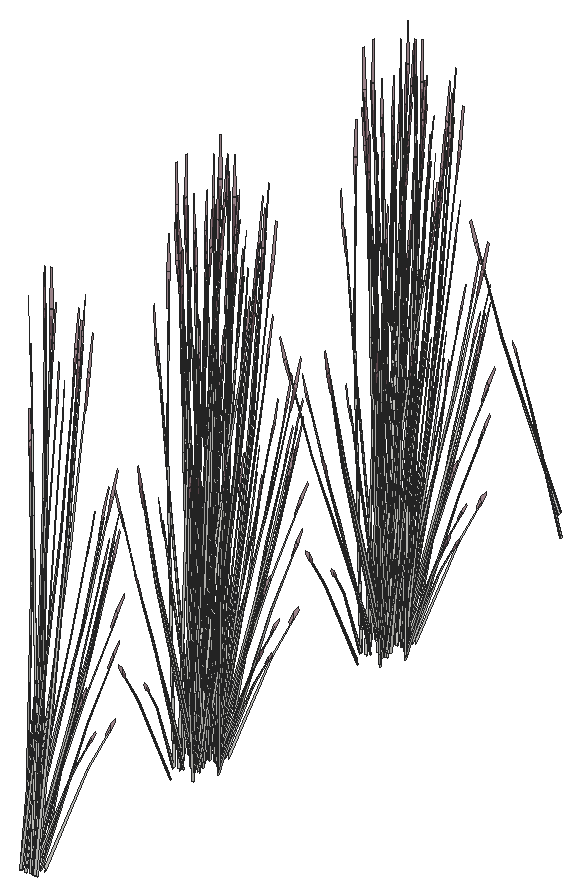
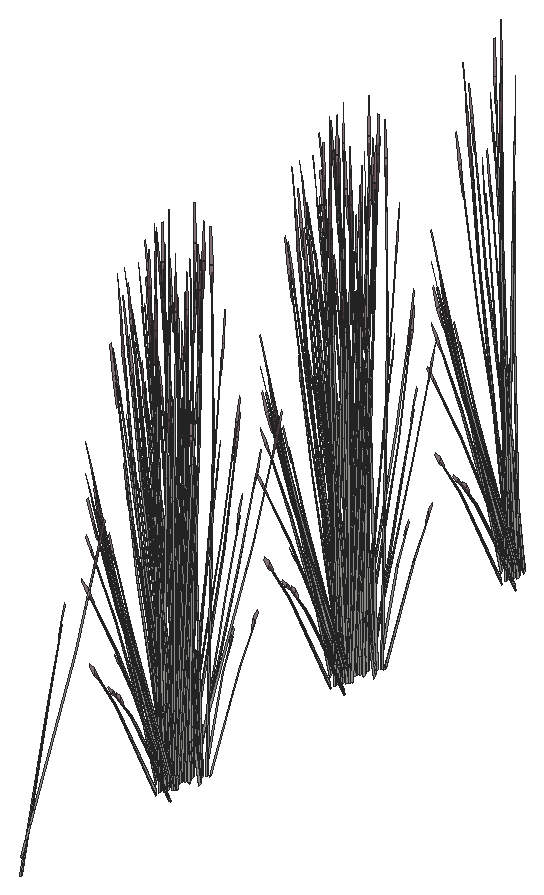
# SketchUp Ruby script. Lengths in inches.
U = 1.inch
M = Sketchup.active_model
def pt(a) = Geom::Point3d.new(a.map { |v| v * U })
def face(e, loops, mat)
  f = e.add_face(loops[0].map { |a| pt(a) })
  loops[1..].each { |l| e.add_face(l.map { |a| pt(a) }).erase! }
  f.material = f.back_material = mat if mat
  f
end
# faces: each face lists its corners as indices into pts; further lists are holes
def faces(e, pts, list, mat = nil) = list.each { |f| face(e, (f[0].is_a?(Array) ? f : [f]).map { |l| l.map { |i| pts[i] } }, mat) }
# xy, xz, yz: faces in a plane at the given z, y or x. An outline is a flat list of corners, or four numbers for a rectangle; further outlines are holes
def ring(l) = l.size == 4 ? [[l[0], l[1]], [l[2], l[1]], [l[2], l[3]], [l[0], l[3]]] : l.each_slice(2).to_a
def flat(e, list, mat, &to3) = list.each { |f| face(e, (f[0].is_a?(Array) ? f : [f]).map { |l| ring(l).map { |u, v| to3.(u, v) } }, mat) }
def xy(e, z, list, mat = nil) = flat(e, list, mat) { |x, y| [x, y, z] }
def xz(e, y, list, mat = nil) = flat(e, list, mat) { |x, z| [x, y, z] }
def yz(e, x, list, mat = nil) = flat(e, list, mat) { |y, z| [x, y, z] }
def lines(e, pts, list) = list.each { |a, b| e.add_line(pt(pts[a]), pt(pts[b])) }
# prism: a flat outline (further loops are holes) pulled along v
def prism(e, loops, v, mat = nil)
  f = face(e, loops, mat); d = Geom::Vector3d.new(v.map { |x| x * U })
  f.pushpull(f.normal.samedirection?(d) ? d.length : -d.length)
end
def box(e, o, s, mat = nil) = prism(e, [[o, [o[0] + s[0], o[1], o[2]], [o[0] + s[0], o[1] + s[1], o[2]], [o[0], o[1] + s[1], o[2]]]], [0, 0, s[2]], mat)
def at(x, y, z, deg = 0) = Geom::Transformation.translation(pt([x, y, z])) * Geom::Transformation.rotation(ORIGIN, Z_AXIS, deg.degrees)
def axes(o, x, y, z) = Geom::Transformation.new([*x, 0, *y, 0, *z, 0, *pt(o).to_a, 1])
def part(name) = M.definitions.add(name)
# library, detail: a bought-in or finely detailed component or shape, given as its bounding box
def library(name, o, s) = part(name).tap { |d| box(d.entities, o, s) }
def detail(e, o, s) = box(e.add_group.entities, o, s)
def put(e, d, t, mat = nil) = e.add_instance(d, t).tap { |i| i.material = mat if mat }
def group(e, t, mat = nil) = e.add_group.tap { |g| g.transformation = t; g.material = mat if mat }.entities
root = M.entities
M.materials.add("LightPink_Translucent").color = [144, 107, 117]
M.materials["LightPink_Translucent"].alpha = 0.75
c1 = part("blade")
p = [[2.15,0.21,22],[0,0.17,0],[0.09,0.45,0],[2.18,0.31,22],[2.29,0.31,22],[0.38,0.45,0],
  [2.48,0.24,33],[2.49,0.24,33],[2.48,0.22,33]]
faces(c1.entities,p,[[0,1,2,3],[4,5,2,3],[6,3,4,7],[8,0,3,6]])
c2 = part("seeds")
p = [[0.3,-0.1,1.38],[-0.01,-0.03,1.59],[-0.01,-0.03,0.03],[0.14,-0.07,-0.07],[0.29,-0.03,3],[0.15,0.01,3.11]]
faces(c2.entities,p,[[0,1,2,3],[1,0,4,5]],"LightPink_Translucent")
c3 = part("blade with seeds")
put(c3.entities,c1,at(0,0,0))
put(c3.entities,c2,axes([2.4,0.25,30.99],[1.5799,-0.05474,1.17369],[-0.12525,1.92788,0.29478],[-0.07173,-0.02425,1.56792]))
put(root,c3,axes([434.57,69.42,0.23],[-0.09062,-0.13571,1.22981],[0.11791,-0.44895,-0.26449],[0.18335,0.06082,0.52581]))
put(root,c3,axes([432.95,69.91,-0.1],[0.37935,0.24773,0],[-0.18257,0.51475,0],[0,0,1.5046]))
put(root,c3,axes([433.02,69.12,0.25],[0.278,0.33153,0.12452],[-0.23189,0.37404,-0.35559],[-0.06454,0.05057,1.09]))
put(root,c3,axes([433.74,69.69,2.28],[0.37615,0.01329,-0.61099],[-0.02526,0.55946,0.07373],[0.15935,0.05904,0.8643]))
put(root,c3,axes([433.32,70.14,0.13],[0.35217,-0.2759,0.427],[0.2105,0.49473,0],[-0.08021,0.06284,1.35453]))
put(root,c3,axes([432.81,69.7,-0.03],[0.1636,0.63392,-0.05171],[-0.46745,0.22213,0],[0.00571,0.02214,1.48069]))
put(root,c3,axes([434.35,68.56,0.04],[0.47052,0,0],[0,0.61671,-0.44382],[0,0.14046,1.40792]))
put(root,c3,axes([434.17,68.87,-0.11],[-0.47029,-0.00441,-0.0428],[0,-0.61671,0.42951],[-0.01478,0.14039,1.36183]))
put(root,c3,axes([433.15,68.34,0.29],[0.42377,0.26329,-0.25022],[-0.20405,0.55571,-0.43002],[0.01332,0.13644,1.37348]))
put(root,c3,axes([433.97,69.92,1.89],[0.2141,0.34548,-0.30456],[-0.24447,0.32704,0.39319],[0.12421,0.04976,0.75234]))
put(root,c3,axes([434.07,68.96,-0.26],[-0.26266,0.34428,-0.26641],[-0.26266,-0.34428,0.26641],[0,0.11089,1.19518]))
put(root,c3,axes([433.1,68.75,-0.1],[-0.18257,0.49721,-0.38476],[-0.37935,-0.23929,0.18517],[0,0.11462,1.23533]))
put(root,c3,axes([433.11,70.17,0],[0.47108,0.17935,0.2645],[-0.11785,0.64108,-0.31383],[-0.07797,0.08023,1.41801]))
put(root,c3,axes([434.25,68.97,-0.26],[0,0.5518,-0.427],[-0.42099,0,0],[0,0.12568,1.35453]))
put(root,c3,axes([433.71,70.12,0.38],[-0.21187,-0.15866,0.9878],[0.27357,-0.16121,0.72577],[0.07379,0.13656,0.21757]))
put(root,c3,axes([433.4,70.52,0.04],[0.23526,0.55293,0],[-0.3936,0.30836,-0.44382],[-0.08964,0.07023,1.40792]))
put(root,c3,axes([433.77,70.71,-0.72],[0.02741,-0.07966,1.51654],[0.34514,-0.23462,-0.23168],[0.10464,0.12143,0.25832]))
put(root,c3,axes([433.32,68.9,-0.2],[0.13798,0.50522,-0.59522],[-0.39745,0.18195,-0.15622],[0.01525,0.17108,1.31385]))
put(root,c3,axes([433.24,70.34,2.03],[0.37131,-0.13117,-0.43945],[0.06495,0.49674,-0.34039],[0.09973,0.14235,0.84085]))
put(root,c3,axes([433.75,70.84,0.29],[-0.2413,-0.01731,0.90352],[0.15935,-0.36755,0.49885],[0.09532,0.13058,0.70873]))
put(root,c3,axes([432.96,69.95,0.23],[0.00664,-0.18292,1.22981],[0.31732,-0.20432,-0.26449],[0.09796,0.21893,0.52581]))
put(root,c3,axes([432.16,70.69,-0.72],[0.0609,-0.03003,1.51654],[0.36632,0.16527,-0.23168],[0.01071,0.18627,0.25832]))
put(root,c3,axes([432.41,70.57,2.03],[0.3699,0.13833,-0.43945],[-0.12679,0.47426,-0.34039],[0.03392,0.19095,0.84085]))
put(root,c3,axes([432.24,70.86,1.89],[-0.11344,0.42434,-0.30456],[-0.33096,-0.12377,0.39319],[0.03035,0.17085,0.75234]))
put(root,c3,axes([432.28,70.48,2.28],[0.17959,0.44867,-0.61099],[-0.36969,0.25004,0.07373],[0.042,0.21679,0.8643]))
put(root,c3,axes([433.22,89.07,0.23],[-0.10696,0.11169,1.22981],[-0.32033,-0.19549,-0.26449],[0.05938,-0.24312,0.52581]))
put(root,c3,axes([432.43,88.47,-0.72],[-0.06312,0.01988,1.51654],[-0.34903,-0.22379,-0.23168],[0.00586,-0.18666,0.25832]))
put(root,c3,axes([433.48,89.9,2.28],[0.00979,-0.51041,-0.61099],[0.4123,0.03428,0.07373],[0.04351,-0.21623,0.8643]))
put(root,c3,axes([432.77,89.08,1.89],[0.11344,-0.42434,-0.30456],[0.33096,0.12377,0.39319],[-0.03035,-0.17085,0.75234]))
put(root,c3,axes([432.83,88.18,0.38],[0.04827,0.32177,0.9878],[-0.26778,-0.17821,0.72577],[0.02882,-0.16476,0.21757]))
put(root,c3,axes([433.4,89.73,2.03],[-0.26937,-0.37076,-0.43945],[0.28456,-0.3247,-0.34039],[0.04099,-0.18838,0.84085]))
put(root,c3,axes([433.65,89.59,1.89],[0.2546,-0.29052,-0.30456],[0.24101,0.33173,0.39319],[0.03667,-0.16855,0.75234]))
put(root,c3,axes([433.97,89.42,-0.72],[-0.05632,-0.04347,1.51654],[-0.14467,-0.48565,-0.23168],[0.09759,-0.13179,0.25832]))
put(root,c3,axes([433.97,90.79,2.28],[0.19655,-0.43539,-0.61099],[0.34443,0.30942,0.07373],[0.11736,-0.15774,0.8643]))
put(root,c3,axes([431.84,89.52,0.04],[-0.23526,-0.55293,0],[0.3936,-0.30836,-0.44382],[0.08964,-0.07023,1.40792]))
put(root,c3,axes([433.96,90.58,2.03],[-0.09666,-0.50384,-0.43945],[0.36608,-0.08814,-0.34039],[0.10491,-0.13533,0.84085]))
put(root,c3,axes([432.16,89.43,-0.26],[0.35217,-0.2759,-0.427],[0.2105,0.49473,0],[0.08021,-0.06284,1.35453]))
put(root,c3,axes([434.25,90.39,0.23],[-0.13443,-0.01634,1.22981],[-0.13772,-0.43844,-0.26449],[0.16514,-0.12403,0.52581]))
put(root,c3,axes([432.58,90.57,-0.23],[0.25345,-0.41475,-0.53624],[0.31485,0.37608,-0.14074],[0.10156,-0.10346,1.18365]))
put(root,c3,axes([434.41,89.58,0.38],[-0.12533,0.28089,0.9878],[-0.10773,-0.37739,0.72577],[0.10352,-0.09457,0.21757]))
put(root,c3,axes([434.23,90.64,1.89],[0.32754,-0.07886,-0.30456],[0.08649,0.45081,0.39319],[0.09386,-0.12109,0.75234]))
put(root,c3,axes([432.14,91.29,-0.1],[0.18257,-0.49721,-0.38476],[0.37935,0.23929,0.18517],[0,-0.11462,1.23533]))
put(root,c3,axes([432.31,91.05,0.29],[-0.04385,-0.62963,-0.25022],[0.45669,-0.03807,-0.43002],[0.08042,-0.08387,1.37348]))
put(root,c3,axes([432.25,89.65,-0.26],[0.35106,0.13653,-0.26641],[-0.08839,0.48081,0.26641],[0.07077,-0.05545,1.19518]))
put(root,c3,axes([432.37,91.54,0.09],[0.42398,0.26744,0.20696],[-0.20405,0.55571,0.43002],[0,-0.1281,1.38067]))
put(root,c3,axes([432.23,91.17,0.34],[-0.40861,0.03406,0.38476],[-0.03695,-0.56543,-0.18517],[0.07315,-0.05731,1.23533]))
put(root,c3,axes([434.13,91.7,2.03],[0.10194,-0.50193,-0.43945],[0.34951,0.17204,-0.34039],[0.14072,-0.04602,0.84085]))
put(root,c3,axes([433.58,89.66,0.04],[0.23526,-0.55293,0],[0.3936,0.30836,-0.44382],[0.08964,0.07023,1.40792]))
put(root,c3,axes([432.22,91.37,0.03],[0.1636,0.61702,0.39349],[-0.46745,0.21456,0.15441],[0.00571,-0.11338,1.36617]))
put(root,c3,axes([434.5,91.84,-0.3],[-0.24235,0.06622,1.21762],[-0.03858,-0.5271,0.0697],[0.16974,-0.07978,0.69287]))
put(root,c3,axes([434.94,91.38,-0.06],[-0.23329,-0.35284,-0.05579],[0.2555,-0.3233,-0.25298],[0.0724,-0.02276,0.83441]))
put(root,c3,axes([432.8,91.42,-0.1],[0,-0.63847,0],[0.47052,0,0],[0,0,1.54332]))
put(root,c3,axes([433.375,89.95,0.13],[-0.35217,-0.2759,0.427],[0.2105,-0.49473,0],[0.08021,0.06284,1.35453]))
put(root,c3,axes([434.0625,91.89,2.28],[0.33065,-0.2437,-0.61099],[0.18427,0.50165,0.07373],[0.15976,-0.05699,0.8643]))
put(root,c3,axes([432.58,91.02,0.03],[-0.312,0.50076,0.39349],[-0.37066,-0.44204,0.15441],[0.07522,-0.04998,1.36617]))
put(root,c3,axes([432.92,91.92,-0.02],[-0.35001,-0.47494,-0.05273],[0.35022,-0.47523,0],[-0.01222,-0.01659,1.50991]))
put(root,c3,axes([432.04,90.2,0.13],[-0.1087,0.54839,0.15172],[-0.39778,-0.15519,0.30174],[0.06871,-0.00267,1.3795]))
put(root,c3,axes([431.875,90.64,-0.63],[-0.37038,0.22092,1.10879],[-0.11789,-0.63387,0.43083],[0.22743,0.01055,1.26112]))
put(root,c3,axes([432.87,90.81,0.25],[0.07259,-0.49245,0.12452],[0.35466,0.08548,-0.35559],[0.06454,0.05057,1.09]))
put(root,c3,axes([434.77,91.5,-0.72],[-0.01967,-0.08377,1.51654],[0.1364,-0.49004,-0.23168],[0.13759,-0.00705,0.25832]))
put(root,c3,axes([432.72,90.9375,0.34],[-0.22605,-0.46315,0.38476],[0.34239,-0.32614,-0.18517],[0.07315,0.05731,1.23533]))
put(root,c3,axes([432,93.02,0.13],[0.40434,-0.14646,0.15172],[0.09984,0.54504,0.30174],[-0.03606,-0.07941,1.3795]))
put(root,c3,axes([432.83,90.97,0.29],[0.37992,-0.36634,-0.25022],[0.25264,0.51764,-0.43002],[0.09374,0.05257,1.37348]))
put(root,c3,axes([434.34,91.93,1.89],[0.31272,0.15393,-0.30456],[-0.09121,0.44909,0.39319],[0.1259,-0.04118,0.75234]))
put(root,c3,axes([433.79,89.99,-0.26],[0.35217,0.2759,-0.427],[-0.2105,0.49473,0],[0.08021,0.06284,1.35453]))
put(root,c3,axes([433.12,91.57,-0.1],[0.42099,0,0],[0,0.57126,0],[0,0,1.5343]))
put(root,c3,axes([433.24,90.23,0.13],[-0.40434,0.14646,0.15172],[-0.09984,-0.54504,0.30174],[0.03606,0.07941,1.3795]))
put(root,c3,axes([433.69,90.2,-0.26],[0.08839,0.48081,-0.26641],[-0.35106,0.13653,0.26641],[0.07077,0.05545,1.19518]))
put(root,c3,axes([432.99,91.28,0.05],[-0.4756,-0.11626,0.42311],[0.09679,-0.6566,0.16603],[0.0695,0.0634,1.46899]))
put(root,c3,axes([432.61,92.9,-0.1],[-0.12277,-0.47573,0],[0.35059,-0.1666,0],[0,0,1.32759]))
put(root,c3,axes([433.07,92.83,-0.12],[0.39505,-0.18722,-0.1651],[0.13882,0.53931,0.00007],[0.04361,-0.02069,1.49552]))
put(root,c3,axes([433.2,93.05,0.13],[0.1087,-0.54839,0.15172],[0.39778,0.15519,0.30174],[-0.06871,0.00267,1.3795]))
put(root,c3,axes([433.11,91.8125,-0.1],[0.26266,0.35642,0],[-0.26266,0.35642,0],[0,0,1.45569]))
put(root,c3,axes([433.82,91.66,0.13],[-0.29564,-0.40194,0.15172],[0.29793,-0.38985,0.30174],[-0.03265,0.08208,1.3795]))
put(root,c3,axes([433.28,91.05,-0.23],[0.39143,0.09047,-0.53624],[-0.0826,0.55804,-0.14074],[0.11681,0.06762,1.18365]))
put(root,c3,axes([435.01,92.02,0.38],[-0.23249,0.0911,0.9878],[0.10944,-0.37648,0.72577],[0.12334,0.02576,0.21757]))
put(root,c3,axes([432.52,93.11,-0.11],[-0.37935,-0.24773,0],[0.18257,-0.51475,0],[0,0,1.39928]))
put(root,c3,axes([433.11,91.39,0.34],[0.18257,-0.49721,0.38476],[0.37935,0.23929,-0.18517],[0,0.11462,1.23533]))
put(root,c3,axes([433.04,91.68,-0.03],[0,0.63816,-0.04848],[-0.47052,0,0],[0,0.02005,1.54256]))
put(root,c3,axes([433.07,91.23,-0.1],[0.22605,0.46315,-0.38476],[-0.34239,0.32614,0.18517],[0.07315,0.05731,1.23533]))
put(root,c3,axes([434.07,91.67,0.13],[0,-0.5518,0.427],[0.42099,0,0],[0,0.12568,1.35453]))
put(root,c3,axes([433.01,92.08,0.34],[0.40861,-0.03406,0.38476],[0.03695,0.56543,-0.18517],[-0.07315,0.05731,1.23533]))
put(root,c3,axes([433.27,91.51,0.25],[0.35059,-0.16092,0.12452],[0.12277,0.45952,-0.35559],[0,0.10113,1.09]))
put(root,c3,axes([434.57,92.63,0.23],[-0.09062,-0.13571,1.22981],[0.11791,-0.44895,-0.26449],[0.18335,0.06082,0.52581]))
put(root,c3,axes([432.95,93.12,-0.1],[0.37935,0.24773,0],[-0.18257,0.51475,0],[0,0,1.5046]))
put(root,c3,axes([433.02,92.33,0.25],[0.278,0.33153,0.12452],[-0.23189,0.37404,-0.35559],[-0.06454,0.05057,1.09]))
put(root,c3,axes([433.74,92.9,2.28],[0.37615,0.01329,-0.61099],[-0.02526,0.55946,0.07373],[0.15935,0.05904,0.8643]))
put(root,c3,axes([433.32,93.35,0.13],[0.35217,-0.2759,0.427],[0.2105,0.49473,0],[-0.08021,0.06284,1.35453]))
put(root,c3,axes([432.81,92.91,-0.03],[0.1636,0.63392,-0.05171],[-0.46745,0.22213,0],[0.00571,0.02214,1.48069]))
put(root,c3,axes([434.35,91.77,0.04],[0.47052,0,0],[0,0.61671,-0.44382],[0,0.14046,1.40792]))
put(root,c3,axes([434.17,92.08,-0.11],[-0.47029,-0.00441,-0.0428],[0,-0.61671,0.42951],[-0.01478,0.14039,1.36183]))
put(root,c3,axes([433.15,91.55,0.29],[0.42377,0.26329,-0.25022],[-0.20405,0.55571,-0.43002],[0.01332,0.13644,1.37348]))
put(root,c3,axes([433.97,93.13,1.89],[0.2141,0.34548,-0.30456],[-0.24447,0.32704,0.39319],[0.12421,0.04976,0.75234]))
put(root,c3,axes([434.07,92.17,-0.26],[-0.26266,0.34428,-0.26641],[-0.26266,-0.34428,0.26641],[0,0.11089,1.19518]))
put(root,c3,axes([433.1,91.96,-0.1],[-0.18257,0.49721,-0.38476],[-0.37935,-0.23929,0.18517],[0,0.11462,1.23533]))
put(root,c3,axes([433.11,93.38,0],[0.47108,0.17935,0.2645],[-0.11785,0.64108,-0.31383],[-0.07797,0.08023,1.41801]))
put(root,c3,axes([434.25,92.18,-0.26],[0,0.5518,-0.427],[-0.42099,0,0],[0,0.12568,1.35453]))
put(root,c3,axes([433.71,93.33,0.38],[-0.21187,-0.15866,0.9878],[0.27357,-0.16121,0.72577],[0.07379,0.13656,0.21757]))
put(root,c3,axes([433.4,93.73,0.04],[0.23526,0.55293,0],[-0.3936,0.30836,-0.44382],[-0.08964,0.07023,1.40792]))
put(root,c3,axes([433.77,93.92,-0.72],[0.02741,-0.07966,1.51654],[0.34514,-0.23462,-0.23168],[0.10464,0.12143,0.25832]))
put(root,c3,axes([433.32,92.11,-0.2],[0.13798,0.50522,-0.59522],[-0.39745,0.18195,-0.15622],[0.01525,0.17108,1.31385]))
put(root,c3,axes([433.24,93.55,2.03],[0.37131,-0.13117,-0.43945],[0.06495,0.49674,-0.34039],[0.09973,0.14235,0.84085]))
put(root,c3,axes([433.75,94.05,0.29],[-0.2413,-0.01731,0.90352],[0.15935,-0.36755,0.49885],[0.09532,0.13058,0.70873]))
put(root,c3,axes([432.96,93.16,0.23],[0.00664,-0.18292,1.22981],[0.31732,-0.20432,-0.26449],[0.09796,0.21893,0.52581]))
put(root,c3,axes([432.16,93.9,-0.72],[0.0609,-0.03003,1.51654],[0.36632,0.16527,-0.23168],[0.01071,0.18627,0.25832]))
put(root,c3,axes([432.41,93.78,2.03],[0.3699,0.13833,-0.43945],[-0.12679,0.47426,-0.34039],[0.03392,0.19095,0.84085]))
put(root,c3,axes([432.24,94.07,1.89],[-0.11344,0.42434,-0.30456],[-0.33096,-0.12377,0.39319],[0.03035,0.17085,0.75234]))
put(root,c3,axes([432.28,93.6875,2.28],[0.17959,0.44867,-0.61099],[-0.36969,0.25004,0.07373],[0.042,0.21679,0.8643]))
put(root,c3,axes([433.22,112.76,0.23],[-0.10696,0.11169,1.22981],[-0.32033,-0.19549,-0.26449],[0.05938,-0.24312,0.52581]))
put(root,c3,axes([432.74,113.15,2.28],[-0.17959,-0.44867,-0.61099],[0.36969,-0.25004,0.07373],[-0.042,-0.21679,0.8643]))
put(root,c3,axes([432.43,112.15,-0.72],[-0.06312,0.01988,1.51654],[-0.34903,-0.22379,-0.23168],[0.00586,-0.18666,0.25832]))
put(root,c3,axes([433.48,113.59,2.28],[0.00979,-0.51041,-0.61099],[0.4123,0.03428,0.07373],[0.04351,-0.21623,0.8643]))
put(root,c3,axes([432.77,112.77,1.89],[0.11344,-0.42434,-0.30456],[0.33096,0.12377,0.39319],[-0.03035,-0.17085,0.75234]))
put(root,c3,axes([432.83,111.87,0.38],[0.04827,0.32177,0.9878],[-0.26778,-0.17821,0.72577],[0.02882,-0.16476,0.21757]))
put(root,c3,axes([433.4,113.42,2.03],[-0.26937,-0.37076,-0.43945],[0.28456,-0.3247,-0.34039],[0.04099,-0.18838,0.84085]))
put(root,c3,axes([433.65,113.28,1.89],[0.2546,-0.29052,-0.30456],[0.24101,0.33173,0.39319],[0.03667,-0.16855,0.75234]))
put(root,c3,axes([433.97,113.11,-0.72],[-0.05632,-0.04347,1.51654],[-0.14467,-0.48565,-0.23168],[0.09759,-0.13179,0.25832]))
put(root,c3,axes([433.97,114.48,2.28],[0.19655,-0.43539,-0.61099],[0.34443,0.30942,0.07373],[0.11736,-0.15774,0.8643]))
put(root,c3,axes([431.84,113.21,0.04],[-0.23526,-0.55293,0],[0.3936,-0.30836,-0.44382],[0.08964,-0.07023,1.40792]))
put(root,c3,axes([433.96,114.27,2.03],[-0.09666,-0.50384,-0.43945],[0.36608,-0.08814,-0.34039],[0.10491,-0.13533,0.84085]))
put(root,c3,axes([432.16,113.125,-0.26],[0.35217,-0.2759,-0.427],[0.2105,0.49473,0],[0.08021,-0.06284,1.35453]))
put(root,c3,axes([434.25,114.08,0.23],[-0.13443,-0.01634,1.22981],[-0.13772,-0.43844,-0.26449],[0.16514,-0.12403,0.52581]))
put(root,c3,axes([432.58,114.25,-0.23],[0.25345,-0.41475,-0.53624],[0.31485,0.37608,-0.14074],[0.10156,-0.10346,1.18365]))
put(root,c3,axes([434.41,113.27,0.38],[-0.12533,0.28089,0.9878],[-0.10773,-0.37739,0.72577],[0.10352,-0.09457,0.21757]))
put(root,c3,axes([434.23,114.33,1.89],[0.32754,-0.07886,-0.30456],[0.08649,0.45081,0.39319],[0.09386,-0.12109,0.75234]))
put(root,c3,axes([432.14,114.98,-0.1],[0.18257,-0.49721,-0.38476],[0.37935,0.23929,0.18517],[0,-0.11462,1.23533]))
put(root,c3,axes([432.31,114.74,0.29],[-0.04385,-0.62963,-0.25022],[0.45669,-0.03807,-0.43002],[0.08042,-0.08387,1.37348]))
put(root,c3,axes([432.25,113.34,-0.26],[0.35106,0.13653,-0.26641],[-0.08839,0.48081,0.26641],[0.07077,-0.05545,1.19518]))
put(root,c3,axes([432.37,115.23,0.09],[0.42398,0.26744,0.20696],[-0.20405,0.55571,0.43002],[0,-0.1281,1.38067]))
put(root,c3,axes([432.23,114.86,0.34],[-0.40861,0.03406,0.38476],[-0.03695,-0.56543,-0.18517],[0.07315,-0.05731,1.23533]))
put(root,c3,axes([434.13,115.39,2.03],[0.10194,-0.50193,-0.43945],[0.34951,0.17204,-0.34039],[0.14072,-0.04602,0.84085]))
put(root,c3,axes([433.58,113.35,0.04],[0.23526,-0.55293,0],[0.3936,0.30836,-0.44382],[0.08964,0.07023,1.40792]))
put(root,c3,axes([432.22,115.06,0.03],[0.1636,0.61702,0.39349],[-0.46745,0.21456,0.15441],[0.00571,-0.11338,1.36617]))
put(root,c3,axes([434.5,115.53,-0.3],[-0.24235,0.06622,1.21762],[-0.03858,-0.5271,0.0697],[0.16974,-0.07978,0.69287]))
put(root,c3,axes([434.94,115.07,-0.06],[-0.23329,-0.35284,-0.05579],[0.2555,-0.3233,-0.25298],[0.0724,-0.02276,0.83441]))
put(root,c3,axes([432.8,115.11,-0.1],[0,-0.63847,0],[0.47052,0,0],[0,0,1.54332]))
put(root,c3,axes([433.375,113.64,0.13],[-0.35217,-0.2759,0.427],[0.2105,-0.49473,0],[0.08021,0.06284,1.35453]))
put(root,c3,axes([434.0625,115.57,2.28],[0.33065,-0.2437,-0.61099],[0.18427,0.50165,0.07373],[0.15976,-0.05699,0.8643]))
put(root,c3,axes([432.58,114.71,0.03],[-0.312,0.50076,0.39349],[-0.37066,-0.44204,0.15441],[0.07522,-0.04998,1.36617]))
put(root,c3,axes([432.92,115.61,-0.02],[-0.35001,-0.47494,-0.05273],[0.35022,-0.47523,0],[-0.01222,-0.01659,1.50991]))
put(root,c3,axes([432.04,113.89,0.13],[-0.1087,0.54839,0.15172],[-0.39778,-0.15519,0.30174],[0.06871,-0.00267,1.3795]))
put(root,c3,axes([431.875,114.33,-0.63],[-0.37038,0.22092,1.10879],[-0.11789,-0.63387,0.43083],[0.22743,0.01055,1.26112]))
put(root,c3,axes([432.87,114.49,0.25],[0.07259,-0.49245,0.12452],[0.35466,0.08548,-0.35559],[0.06454,0.05057,1.09]))
put(root,c3,axes([434.77,115.1875,-0.72],[-0.01967,-0.08377,1.51654],[0.1364,-0.49004,-0.23168],[0.13759,-0.00705,0.25832]))
put(root,c3,axes([432.72,114.625,0.34],[-0.22605,-0.46315,0.38476],[0.34239,-0.32614,-0.18517],[0.07315,0.05731,1.23533]))
put(root,c3,axes([432,116.71,0.13],[0.40434,-0.14646,0.15172],[0.09984,0.54504,0.30174],[-0.03606,-0.07941,1.3795]))
put(root,c3,axes([432.83,114.65,0.29],[0.37992,-0.36634,-0.25022],[0.25264,0.51764,-0.43002],[0.09374,0.05257,1.37348]))
put(root,c3,axes([434.34,115.62,1.89],[0.31272,0.15393,-0.30456],[-0.09121,0.44909,0.39319],[0.1259,-0.04118,0.75234]))
put(root,c3,axes([433.79,113.68,-0.26],[0.35217,0.2759,-0.427],[-0.2105,0.49473,0],[0.08021,0.06284,1.35453]))
put(root,c3,axes([433.12,115.25,-0.1],[0.42099,0,0],[0,0.57126,0],[0,0,1.5343]))
put(root,c3,axes([433.24,113.92,0.13],[-0.40434,0.14646,0.15172],[-0.09984,-0.54504,0.30174],[0.03606,0.07941,1.3795]))
put(root,c3,axes([433.69,113.89,-0.26],[0.08839,0.48081,-0.26641],[-0.35106,0.13653,0.26641],[0.07077,0.05545,1.19518]))
put(root,c3,axes([432.99,114.96,0.05],[-0.4756,-0.11626,0.42311],[0.09679,-0.6566,0.16603],[0.0695,0.0634,1.46899]))
put(root,c3,axes([432.61,116.59,-0.1],[-0.12277,-0.47573,0],[0.35059,-0.1666,0],[0,0,1.32759]))
put(root,c3,axes([433.07,116.52,-0.12],[0.39505,-0.18722,-0.1651],[0.13882,0.53931,0.00007],[0.04361,-0.02069,1.49552]))
put(root,c3,axes([433.2,116.74,0.13],[0.1087,-0.54839,0.15172],[0.39778,0.15519,0.30174],[-0.06871,0.00267,1.3795]))
put(root,c3,axes([433.11,115.5,-0.1],[0.26266,0.35642,0],[-0.26266,0.35642,0],[0,0,1.45569]))
put(root,c3,axes([433.82,115.34,0.13],[-0.29564,-0.40194,0.15172],[0.29793,-0.38985,0.30174],[-0.03265,0.08208,1.3795]))
put(root,c3,axes([433.28,114.74,-0.23],[0.39143,0.09047,-0.53624],[-0.0826,0.55804,-0.14074],[0.11681,0.06762,1.18365]))
put(root,c3,axes([435.01,115.71,0.38],[-0.23249,0.0911,0.9878],[0.10944,-0.37648,0.72577],[0.12334,0.02576,0.21757]))
put(root,c3,axes([432.52,116.8,-0.11],[-0.37935,-0.24773,0],[0.18257,-0.51475,0],[0,0,1.39928]))
put(root,c3,axes([433.11,115.08,0.34],[0.18257,-0.49721,0.38476],[0.37935,0.23929,-0.18517],[0,0.11462,1.23533]))
put(root,c3,axes([433.04,115.37,-0.03],[0,0.63816,-0.04848],[-0.47052,0,0],[0,0.02005,1.54256]))
put(root,c3,axes([433.07,114.91,-0.1],[0.22605,0.46315,-0.38476],[-0.34239,0.32614,0.18517],[0.07315,0.05731,1.23533]))
put(root,c3,axes([434.07,115.36,0.13],[0,-0.5518,0.427],[0.42099,0,0],[0,0.12568,1.35453]))
put(root,c3,axes([433.01,115.77,0.34],[0.40861,-0.03406,0.38476],[0.03695,0.56543,-0.18517],[-0.07315,0.05731,1.23533]))
put(root,c3,axes([433.27,115.2,0.25],[0.35059,-0.16092,0.12452],[0.12277,0.45952,-0.35559],[0,0.10113,1.09]))
put(root,c3,axes([434.57,116.32,0.23],[-0.09062,-0.13571,1.22981],[0.11791,-0.44895,-0.26449],[0.18335,0.06082,0.52581]))
put(root,c3,axes([432.95,116.81,-0.1],[0.37935,0.24773,0],[-0.18257,0.51475,0],[0,0,1.5046]))
put(root,c3,axes([433.02,116.02,0.25],[0.278,0.33153,0.12452],[-0.23189,0.37404,-0.35559],[-0.06454,0.05057,1.09]))
put(root,c3,axes([433.74,116.59,2.28],[0.37615,0.01329,-0.61099],[-0.02526,0.55946,0.07373],[0.15935,0.05904,0.8643]))
put(root,c3,axes([433.32,117.04,0.13],[0.35217,-0.2759,0.427],[0.2105,0.49473,0],[-0.08021,0.06284,1.35453]))
put(root,c3,axes([432.81,116.6,-0.03],[0.1636,0.63392,-0.05171],[-0.46745,0.22213,0],[0.00571,0.02214,1.48069]))
put(root,c3,axes([434.35,115.45,0.04],[0.47052,0,0],[0,0.61671,-0.44382],[0,0.14046,1.40792]))
put(root,c3,axes([434.17,115.77,-0.11],[-0.47029,-0.00441,-0.0428],[0,-0.61671,0.42951],[-0.01478,0.14039,1.36183]))
put(root,c3,axes([433.15,115.23,0.29],[0.42377,0.26329,-0.25022],[-0.20405,0.55571,-0.43002],[0.01332,0.13644,1.37348]))
put(root,c3,axes([433.97,116.82,1.89],[0.2141,0.34548,-0.30456],[-0.24447,0.32704,0.39319],[0.12421,0.04976,0.75234]))
put(root,c3,axes([434.07,115.86,-0.26],[-0.26266,0.34428,-0.26641],[-0.26266,-0.34428,0.26641],[0,0.11089,1.19518]))
put(root,c3,axes([433.1,115.65,-0.1],[-0.18257,0.49721,-0.38476],[-0.37935,-0.23929,0.18517],[0,0.11462,1.23533]))
put(root,c3,axes([433.11,117.07,0],[0.47108,0.17935,0.2645],[-0.11785,0.64108,-0.31383],[-0.07797,0.08023,1.41801]))
put(root,c3,axes([434.25,115.87,-0.26],[0,0.5518,-0.427],[-0.42099,0,0],[0,0.12568,1.35453]))
put(root,c3,axes([433.71,117.02,0.38],[-0.21187,-0.15866,0.9878],[0.27357,-0.16121,0.72577],[0.07379,0.13656,0.21757]))
put(root,c3,axes([433.4,117.42,0.04],[0.23526,0.55293,0],[-0.3936,0.30836,-0.44382],[-0.08964,0.07023,1.40792]))
put(root,c3,axes([433.77,117.61,-0.72],[0.02741,-0.07966,1.51654],[0.34514,-0.23462,-0.23168],[0.10464,0.12143,0.25832]))
put(root,c3,axes([433.32,115.8,-0.2],[0.13798,0.50522,-0.59522],[-0.39745,0.18195,-0.15622],[0.01525,0.17108,1.31385]))
put(root,c3,axes([433.24,117.24,2.03],[0.37131,-0.13117,-0.43945],[0.06495,0.49674,-0.34039],[0.09973,0.14235,0.84085]))
put(root,c3,axes([433.75,117.74,0.29],[-0.2413,-0.01731,0.90352],[0.15935,-0.36755,0.49885],[0.09532,0.13058,0.70873]))
put(root,c3,axes([432.96,116.85,0.23],[0.00664,-0.18292,1.22981],[0.31732,-0.20432,-0.26449],[0.09796,0.21893,0.52581]))
put(root,c3,axes([432.16,117.59,-0.72],[0.0609,-0.03003,1.51654],[0.36632,0.16527,-0.23168],[0.01071,0.18627,0.25832]))
put(root,c3,axes([432.41,117.47,2.03],[0.3699,0.13833,-0.43945],[-0.12679,0.47426,-0.34039],[0.03392,0.19095,0.84085]))
put(root,c3,axes([432.24,117.76,1.89],[-0.11344,0.42434,-0.30456],[-0.33096,-0.12377,0.39319],[0.03035,0.17085,0.75234]))
put(root,c3,axes([432.28,117.375,2.28],[0.17959,0.44867,-0.61099],[-0.36969,0.25004,0.07373],[0.042,0.21679,0.8643]))
put(root,c3,axes([433.22,136.87,0.23],[-0.10696,0.11169,1.22981],[-0.32033,-0.19549,-0.26449],[0.05938,-0.24312,0.52581]))
put(root,c3,axes([432.74,137.26,2.28],[-0.17959,-0.44867,-0.61099],[0.36969,-0.25004,0.07373],[-0.042,-0.21679,0.8643]))
